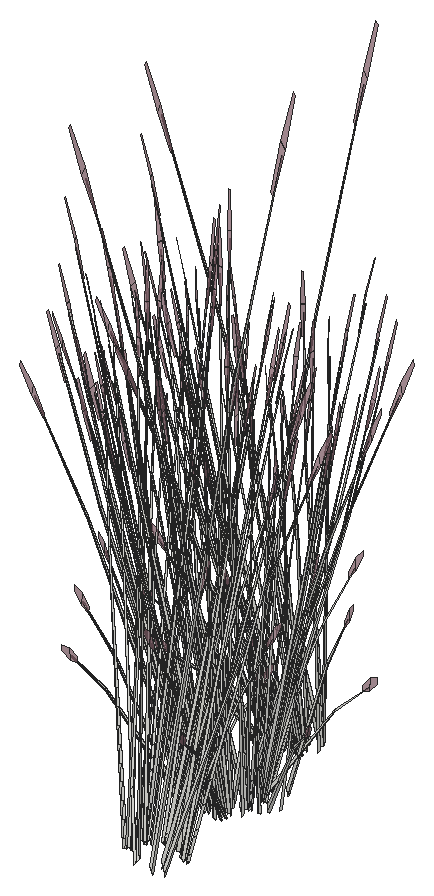
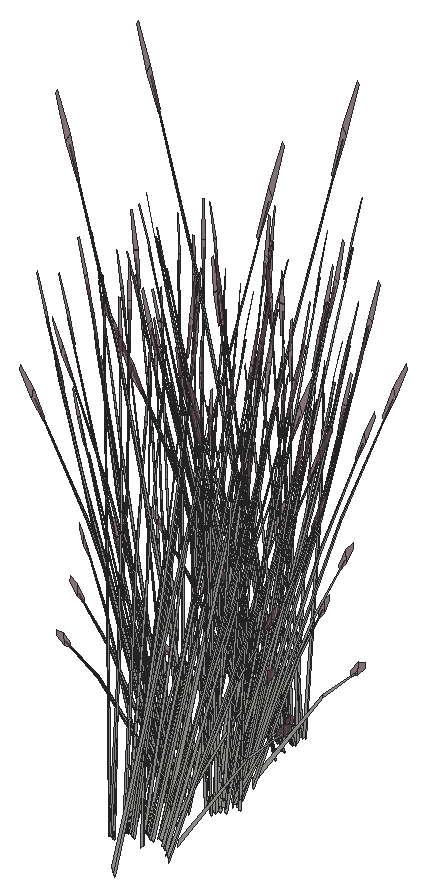
# SketchUp Ruby script. Lengths in inches.
U = 1.inch
M = Sketchup.active_model
def pt(a) = Geom::Point3d.new(a.map { |v| v * U })
def face(e, loops, mat)
  f = e.add_face(loops[0].map { |a| pt(a) })
  loops[1..].each { |l| e.add_face(l.map { |a| pt(a) }).erase! }
  f.material = f.back_material = mat if mat
  f
end
# faces: each face lists its corners as indices into pts; further lists are holes
def faces(e, pts, list, mat = nil) = list.each { |f| face(e, (f[0].is_a?(Array) ? f : [f]).map { |l| l.map { |i| pts[i] } }, mat) }
# xy, xz, yz: faces in a plane at the given z, y or x. An outline is a flat list of corners, or four numbers for a rectangle; further outlines are holes
def ring(l) = l.size == 4 ? [[l[0], l[1]], [l[2], l[1]], [l[2], l[3]], [l[0], l[3]]] : l.each_slice(2).to_a
def flat(e, list, mat, &to3) = list.each { |f| face(e, (f[0].is_a?(Array) ? f : [f]).map { |l| ring(l).map { |u, v| to3.(u, v) } }, mat) }
def xy(e, z, list, mat = nil) = flat(e, list, mat) { |x, y| [x, y, z] }
def xz(e, y, list, mat = nil) = flat(e, list, mat) { |x, z| [x, y, z] }
def yz(e, x, list, mat = nil) = flat(e, list, mat) { |y, z| [x, y, z] }
def lines(e, pts, list) = list.each { |a, b| e.add_line(pt(pts[a]), pt(pts[b])) }
# prism: a flat outline (further loops are holes) pulled along v
def prism(e, loops, v, mat = nil)
  f = face(e, loops, mat); d = Geom::Vector3d.new(v.map { |x| x * U })
  f.pushpull(f.normal.samedirection?(d) ? d.length : -d.length)
end
def box(e, o, s, mat = nil) = prism(e, [[o, [o[0] + s[0], o[1], o[2]], [o[0] + s[0], o[1] + s[1], o[2]], [o[0], o[1] + s[1], o[2]]]], [0, 0, s[2]], mat)
def at(x, y, z, deg = 0) = Geom::Transformation.translation(pt([x, y, z])) * Geom::Transformation.rotation(ORIGIN, Z_AXIS, deg.degrees)
def axes(o, x, y, z) = Geom::Transformation.new([*x, 0, *y, 0, *z, 0, *pt(o).to_a, 1])
def part(name) = M.definitions.add(name)
# library, detail: a bought-in or finely detailed component or shape, given as its bounding box
def library(name, o, s) = part(name).tap { |d| box(d.entities, o, s) }
def detail(e, o, s) = box(e.add_group.entities, o, s)
def put(e, d, t, mat = nil) = e.add_instance(d, t).tap { |i| i.material = mat if mat }
def group(e, t, mat = nil) = e.add_group.tap { |g| g.transformation = t; g.material = mat if mat }.entities
root = M.entities
M.materials.add("LightPink_Translucent").color = [144, 107, 117]
M.materials["LightPink_Translucent"].alpha = 0.75
c1 = part("blade")
p = [[2.15,0.21,22],[0,0.17,0],[0.09,0.45,0],[2.18,0.31,22],[2.29,0.31,22],[0.38,0.45,0],
  [2.48,0.24,33],[2.49,0.24,33],[2.48,0.22,33]]
faces(c1.entities,p,[[0,1,2,3],[4,5,2,3],[6,3,4,7],[8,0,3,6]])
c2 = part("seeds")
p = [[0.3,-0.1,1.38],[-0.01,-0.03,1.59],[-0.01,-0.03,0.03],[0.14,-0.07,-0.07],[0.29,-0.03,3],[0.15,0.01,3.11]]
faces(c2.entities,p,[[0,1,2,3],[1,0,4,5]],"LightPink_Translucent")
c3 = part("blade with seeds")
put(c3.entities,c1,at(0,0,0))
put(c3.entities,c2,axes([2.4,0.25,30.99],[1.5799,-0.05474,1.17369],[-0.12525,1.92788,0.29478],[-0.07173,-0.02425,1.56792]))
put(root,c3,axes([430.69,389.83,153.82],[0.23317,0.29531,-0.29918],[-0.26625,0.27955,0.38624],[0.13527,0.04253,0.73904]))
put(root,c3,axes([430.57,389.94,154],[-0.02064,0.35866,0.05432],[-0.3116,-0.00983,0.42765],[0.11936,0.03753,0.65209]))
put(root,c3,axes([428,395.12,154.21],[-0.19559,-0.38351,-0.60019],[0.40262,-0.21373,0.07243],[-0.04574,-0.1853,0.84903]))
put(root,c3,axes([427.23,389.3,153.82],[-0.35672,0.06741,-0.29918],[-0.09419,-0.38534,0.38624],[-0.10222,0.1035,0.73904]))
put(root,c3,axes([430.6,389.83,154],[-0.30217,0.31079,0.40553],[-0.2606,-0.33005,0.33437],[0.14177,0.05733,0.83914]))
put(root,c3,axes([428.8125,395.49,154.21],[0.01066,-0.43628,-0.60019],[0.44902,0.0293,0.07243],[0.04739,-0.18483,0.84903]))
put(root,c3,axes([429.4375,394.8125,153.98],[-0.00396,-0.09387,1.47793],[-0.33411,-0.2713,-0.23373],[0.05166,-0.16446,0.11853]))
put(root,c3,axes([428.03,394.79,153.82],[0.12355,-0.36271,-0.29918],[0.36044,0.10579,0.38624],[-0.03305,-0.14603,0.73904]))
put(root,c3,axes([428.31,395.27,153.27],[-0.0763,0.16212,1.44779],[-0.3201,-0.3355,0.11706],[0.1444,-0.2091,0.61892]))
put(root,c3,axes([429.35,394.48,153.98],[-0.04162,0.03603,1.49853],[-0.40776,-0.12155,-0.1416],[-0.01476,-0.15722,0.26519]))
put(root,c3,axes([429.86,389.07,153.27],[-0.15222,-0.08126,1.44779],[0.31502,-0.34091,0.11706],[0.19634,0.15379,0.61892]))
put(root,c3,axes([429.88,388,153.78],[-0.35411,-0.24507,1.16821],[0.37391,-0.38156,0.50405],[0.11425,0.22994,1.12919]))
put(root,c3,axes([427.85,395.04,153.95],[-0.40284,-0.11824,-0.43168],[0.13808,-0.40538,-0.33437],[-0.03694,-0.16321,0.82598]))
put(root,c3,axes([427.33,389.04,154.25],[0.37908,0.26007,-0.10273],[-0.21839,0.37663,-0.57019],[-0.1071,0.13092,0.8664]))
put(root,c3,axes([429.61,390.39,154.25],[0.2442,-0.40372,-0.10273],[0.35364,0.23259,-0.57019],[0.12293,0.11406,0.8664]))
put(root,c3,axes([428.72,395.35,153.95],[-0.29336,-0.31691,-0.43168],[0.3099,-0.27755,-0.33437],[0.04464,-0.16102,0.82598]))
put(root,c3,axes([427.13,393.78,153.98],[-0.00765,0.05653,1.49853],[-0.37706,0.20517,-0.1416],[-0.11096,-0.10488,0.26519]))
put(root,c3,axes([427.84,388.92,153.27],[0.10236,-0.14492,1.44779],[0.25844,0.39118,0.11706],[-0.17726,0.17814,0.61892]))
put(root,c3,axes([427.52,389.35,153.95],[0.10528,0.43067,-0.43168],[-0.39868,0.07534,-0.33437],[-0.11425,0.11568,0.82598]))
put(root,c3,axes([429.29,390.72,153.98],[0.00121,-0.0571,1.49853],[0.35119,-0.25193,-0.1416],[0.12199,0.08992,0.26519]))
put(root,c3,axes([427.75,390.07,154],[-0.33677,-0.02198,0.05432],[0.00923,-0.33185,0.42765],[-0.03524,0.12712,0.65209]))
put(root,c3,axes([428.19,395.02,154.25],[-0.40102,0.2196,-0.10273],[-0.19707,-0.38974,-0.57019],[-0.05291,-0.16424,0.8664]))
put(root,c3,axes([429.03,395.52,154.25],[-0.45039,-0.02337,-0.10273],[0.01231,-0.44247,-0.57019],[0.03129,-0.17041,0.8664]))
put(root,c3,axes([427.85,390.1,154],[-0.29182,-0.32181,0.40553],[0.3099,-0.27755,0.33437],[-0.05383,0.15098,0.83914]))
put(root,c3,axes([429.9,390.18,153.95],[0.40438,-0.11212,-0.43168],[0.07074,0.4246,-0.33437],[0.10862,0.12168,0.82598]))
put(root,c3,axes([429,395.23,153.82],[0.27728,-0.24833,-0.29918],[0.26248,0.28355,0.38624],[0.03994,-0.14407,0.73904]))
put(root,c3,axes([428.19,394.85,154],[0.30197,-0.1603,0.05432],[0.1478,0.29231,0.42765],[-0.02916,-0.12885,0.65209]))
put(root,c3,axes([427.12,395.23,154.21],[-0.34944,-0.22798,-0.60019],[0.24834,-0.39949,0.07243],[-0.1266,-0.13612,0.84903]))
put(root,c3,axes([426.99,394.93,153.82],[-0.06329,-0.37991,-0.29918],[0.36182,-0.10032,0.38624],[-0.09718,-0.10887,0.73904]))
put(root,c3,axes([429.7,390.53,154],[-0.18625,0.29962,0.05432],[-0.26523,-0.17444,0.42765],[0.08575,0.09606,0.65209]))
put(root,c3,axes([427.15,394.89,154],[0.18625,-0.29962,0.05432],[0.26523,0.17444,0.42765],[-0.08575,-0.09606,0.65209]))
put(root,c3,axes([429.78,390.45,154],[-0.4076,0.10824,0.40553],[-0.07074,-0.4246,0.33437],[0.09586,0.12514,0.83914]))
put(root,c3,axes([426.22,395.48,153.27],[0.15222,0.08126,1.44779],[-0.31502,0.34091,0.11706],[-0.19634,-0.15379,0.61892]))
put(root,c3,axes([427.77,389.28,153.27],[0.0763,-0.16212,1.44779],[0.3201,0.3355,0.11706],[-0.1444,0.2091,0.61892]))
put(root,c3,axes([428.66,390.58,154],[-0.30197,0.1603,0.05432],[-0.1478,-0.29231,0.42765],[0.02916,0.12885,0.65209]))
put(root,c3,axes([427.85,390.19,153.82],[-0.27728,0.24833,-0.29918],[-0.26248,-0.28355,0.38624],[-0.03994,0.14407,0.73904]))
put(root,c3,axes([426.9,390.12,153.98],[-0.01019,0.09334,1.47793],[0.28908,0.3247,-0.23373],[-0.07568,0.15355,0.11853]))
put(root,c3,axes([426.95,395.24,153.95],[-0.40438,0.11212,-0.43168],[-0.07074,-0.4246,-0.33437],[-0.10862,-0.12168,0.82598]))
put(root,c3,axes([427.82,389.91,154.56],[0.45039,0.02337,-0.11403],[-0.01231,0.44247,-0.63292],[-0.03129,0.17041,0.9617]))
put(root,c3,axes([428.66,390.4,154.25],[0.40102,-0.2196,-0.10273],[0.19707,0.38974,-0.57019],[0.05291,0.16424,0.8664]))
put(root,c3,axes([427.23,394.86,154.59],[-0.2735,0.45217,-0.11506],[-0.39608,-0.2605,-0.63862],[-0.13768,-0.12775,0.97037]))
put(root,c3,axes([429.1,395.36,154],[0.33677,0.02198,0.05432],[-0.00923,0.33185,0.42765],[0.03524,-0.12712,0.65209]))
put(root,c3,axes([429.34,396.25,154.21],[0.21406,-0.37215,-0.60019],[0.37511,0.26448,0.07243],[0.12781,-0.13483,0.84903]))
put(root,c3,axes([429.33,396.08,153.95],[-0.10528,-0.43067,-0.43168],[0.39868,-0.07534,-0.33437],[0.11425,-0.11568,0.82598]))
put(root,c3,axes([428.13,390.07,154.23],[0.29336,0.31691,-0.47917],[-0.3099,0.27755,-0.37115],[-0.04464,0.16102,0.91684]))
put(root,c3,axes([426.1875,394.73,153.98],[-0.08817,-0.00333,1.47793],[-0.28072,0.33293,-0.23373],[-0.14978,-0.06803,0.11853]))
put(root,c3,axes([429.52,396.39,154.25],[-0.37908,-0.26007,-0.10273],[0.21839,-0.37663,-0.57019],[0.1071,-0.13092,0.8664]))
put(root,c3,axes([429,390.38,153.95],[0.40284,0.11824,-0.43168],[-0.13808,0.40538,-0.33437],[0.03694,0.16321,0.82598]))
put(root,c3,axes([429.23,389.55,153.27],[-0.09368,-0.15143,1.44779],[0.43286,-0.12749,0.11706],[0.09783,0.23774,0.61892]))
put(root,c3,axes([427.95,397.81,152.81],[0.35414,0.19019,1.27785],[-0.34693,0.40974,0.50532],[-0.1554,-0.24285,1.07126]))
put(root,c3,axes([428.82,390.63,153.82],[-0.12355,0.36271,-0.29918],[-0.36044,-0.10579,0.38624],[0.03305,0.14603,0.73904]))
put(root,c3,axes([428.04,389.93,154.51],[-0.01066,0.43628,-0.66621],[-0.44902,-0.0293,0.0804],[-0.04739,0.18483,0.94242]))
put(root,c3,axes([430.45,396.27,153.98],[-0.05353,-0.00358,1.49853],[-0.22227,-0.38383,-0.1416],[0.08926,-0.1262,0.26519]))
put(root,c3,axes([426.87,391.08,153.98],[0.04649,-0.02848,1.49853],[0.38427,0.18941,-0.1416],[-0.00903,0.15771,0.26519]))
put(root,c3,axes([428.46,389.62,153.27],[-0.01003,-0.18103,1.44779],[0.43473,0.12009,0.11706],[-0.02689,0.25798,0.61892]))
put(root,c3,axes([429.625,396.125,153.82],[0.35672,-0.06741,-0.29918],[0.09419,0.38534,0.38624],[0.10222,-0.1035,0.73904]))
put(root,c3,axes([428.85,390.31,154.21],[0.19559,0.38351,-0.60019],[-0.40262,0.21373,0.07243],[0.04574,0.1853,0.84903]))
put(root,c3,axes([426.28,395.48,154],[0.02064,-0.35866,0.05432],[0.3116,0.00983,0.42765],[-0.11936,-0.03753,0.65209]))
put(root,c3,axes([426.16,395.59,153.82],[-0.23317,-0.29531,-0.29918],[0.26625,-0.27955,0.38624],[-0.13527,-0.04253,0.73904]))
put(root,c3,axes([428.5625,391.27,153.98],[0.05195,0.07595,1.47793],[0.41921,0.02984,-0.23373],[0.04216,0.1675,0.11853]))
put(root,c3,axes([426.4,395.79,154.21],[-0.40965,-0.01136,-0.60019],[0.02751,-0.47821,0.07243],[-0.17355,-0.05047,0.84903]))
put(root,c3,axes([427.89,390.54,152.84],[0.009,-0.24349,1.30391],[0.40497,0.12861,0.18019],[-0.03509,0.2595,0.61571]))
put(root,c3,axes([429.66,396.29,154],[0.28133,0.19836,0.05432],[-0.16379,0.28248,0.42765],[0.0902,-0.09132,0.65209]))
put(root,c3,axes([430.65,396.73,153.98],[0.05687,-0.07184,1.47793],[-0.07279,-0.44069,-0.23373],[0.14268,-0.08356,0.11853]))
put(root,c3,axes([425.85,395.01,153.98],[0.03038,0.04707,1.49853],[-0.14646,0.42312,-0.1416],[-0.14833,0.00306,0.26519]))
put(root,c3,axes([426.27,395.89,153.95],[-0.29757,0.31243,-0.43168],[-0.2606,-0.33005,-0.33437],[-0.15119,-0.04754,0.82598]))
put(root,c3,axes([426.42,395.56,154.25],[-0.02194,0.47967,-0.10273],[-0.41546,-0.01311,-0.57019],[-0.16001,-0.03332,0.8664]))
put(root,c3,axes([429.53,397.4,154.25],[-0.20619,-0.42709,-0.10273],[0.36595,-0.20988,-0.57019],[0.15422,-0.05635,0.8664]))
put(root,c3,axes([429.51,397.03,153.95],[0.11102,-0.42903,-0.43168],[0.38064,0.14706,-0.33437],[0.15325,-0.03934,0.82598]))
put(root,c3,axes([425.89,396.22,153.27],[0.16998,-0.01068,1.44779],[-0.11276,0.46299,0.11706],[-0.24224,-0.02864,0.61892]))
put(root,c3,axes([429.44,397.19,154.21],[0.3601,-0.20831,-0.60019],[0.20068,0.4288,0.07243],[0.17399,-0.04871,0.84903]))
put(root,c3,axes([425.8,396.46,154],[-0.15051,-0.3216,0.05432],[0.27447,-0.15741,0.42765],[-0.12099,0.03106,0.65209]))
put(root,c3,axes([429.75,397.23,153.82],[0.34057,0.13158,-0.29918],[-0.09933,0.38387,0.38624],[0.13712,-0.0352,0.73904]))
put(root,c3,axes([425.74,396.62,153.82],[-0.34057,-0.13158,-0.29918],[0.09933,-0.38387,0.38624],[-0.13712,0.0352,0.73904]))
put(root,c3,axes([428.82,396.75,153.27],[-0.16998,0.01068,1.44779],[0.11276,-0.46299,0.11706],[0.24224,0.02864,0.61892]))
put(root,c3,axes([429.7,397.39,154],[0.15051,0.3216,0.05432],[-0.27447,0.15741,0.42765],[0.12099,-0.03106,0.65209]))
put(root,c3,axes([426.78,396.55,152.82],[0.11649,-0.06823,1.49584],[0.04017,0.47639,0.11706],[-0.25231,0.06321,0.53462]))
put(root,c3,axes([430.35,398.67,153.98],[-0.03706,-0.04129,1.49853],[0.08106,-0.44261,-0.1416],[0.14596,-0.02828,0.26519]))
put(root,c3,axes([425.53,396.875,153.98],[-0.06692,0.06124,1.47793],[0.00569,0.44742,-0.23373],[-0.15339,0.05818,0.11853]))
put(root,c3,axes([425.98,396.8125,153.95],[-0.11102,0.42903,-0.43168],[-0.38064,-0.14706,-0.33437],[-0.15325,0.03934,0.82598]))
put(root,c3,axes([425.96,396.45,154.25],[0.20619,0.42709,-0.10273],[-0.36595,0.20988,-0.57019],[-0.15422,0.05635,0.8664]))
put(root,c3,axes([430.03,398.3,153.32],[-0.07843,-0.39649,-0.0295],[0.37072,-0.09115,-0.13375],[0.07742,0.02514,0.44114]))
put(root,c3,axes([429.07,398.29,154.25],[0.02194,-0.47967,-0.10273],[0.41546,0.01311,-0.57019],[0.16001,0.03332,0.8664]))
put(root,c3,axes([425.76,402.58,153.27],[0.09368,0.15143,1.44779],[-0.43286,0.12749,0.11706],[-0.09783,-0.23774,0.61892]))
put(root,c3,axes([426.47,401.58,153.98],[-0.06268,-0.06613,1.47793],[-0.4183,0.04193,-0.23373],[-0.06676,-0.15817,0.11853]))
put(root,c3,axes([426.91,402.7,154.21],[-0.19559,-0.38351,-0.60019],[0.40262,-0.21373,0.07243],[-0.04574,-0.1853,0.84903]))
put(root,c3,axes([429.43,398,153.98],[0.08791,-0.00798,1.47793],[0.24113,-0.36643,-0.23373],[0.15637,0.04837,0.11853]))
put(root,c3,axes([425.84,397.56,154],[-0.28133,-0.19836,0.05432],[0.16379,-0.28248,0.42765],[-0.0902,0.09132,0.65209]))
put(root,c3,axes([425.97,397.04,153.27],[0.14219,-0.09977,1.44779],[0.11971,0.461,0.11706],[-0.22323,0.10419,0.61892]))
put(root,c3,axes([429.09,398.06,154.21],[0.40965,0.01136,-0.60019],[-0.02751,0.47821,0.07243],[0.17355,0.05047,0.84903]))
put(root,c3,axes([427.73,403.07,154.21],[0.01066,-0.43628,-0.60019],[0.44902,0.0293,0.07243],[0.04739,-0.18483,0.84903]))
put(root,c3,axes([428.35,402.39,153.98],[-0.00396,-0.09387,1.47793],[-0.33411,-0.2713,-0.23373],[0.05166,-0.16446,0.11853]))
put(root,c3,axes([426.95,402.37,153.82],[0.12355,-0.36271,-0.29918],[0.36044,0.10579,0.38624],[-0.03305,-0.14603,0.73904]))
put(root,c3,axes([427.22,402.85,153.27],[-0.0763,0.16212,1.44779],[-0.3201,-0.3355,0.11706],[0.1444,-0.2091,0.61892]))
put(root,c3,axes([428.26,402.05,153.98],[-0.04162,0.03603,1.49853],[-0.40776,-0.12155,-0.1416],[-0.01476,-0.15722,0.26519]))
put(root,c3,axes([426.77,402.62,153.95],[-0.40284,-0.11824,-0.43168],[0.13808,-0.40538,-0.33437],[-0.03694,-0.16321,0.82598]))
put(root,c3,axes([424.79,397.33,153.98],[0.0523,0.01265,1.49853],[0.16179,0.41674,-0.1416],[-0.10706,0.10938,0.26519]))
put(root,c3,axes([427.64,402.93,153.95],[-0.29336,-0.31691,-0.43168],[0.3099,-0.27755,-0.33437],[0.04464,-0.16102,0.82598]))
put(root,c3,axes([429.34,398.26,153.82],[0.23317,0.29531,-0.29918],[-0.26625,0.27955,0.38624],[0.13527,0.04253,0.73904]))
put(root,c3,axes([429.22,398.37,154],[-0.02064,0.35866,0.05432],[-0.3116,-0.00983,0.42765],[0.11936,0.03753,0.65209]))
put(root,c3,axes([426.04,401.36,153.98],[-0.00765,0.05653,1.49853],[-0.37706,0.20517,-0.1416],[-0.11096,-0.10488,0.26519]))
put(root,c3,axes([425.87,397.73,153.82],[-0.35672,0.06741,-0.29918],[-0.09419,-0.38534,0.38624],[-0.10222,0.1035,0.73904]))
put(root,c3,axes([427.11,402.6,154.25],[-0.40102,0.2196,-0.10273],[-0.19707,-0.38974,-0.57019],[-0.05291,-0.16424,0.8664]))
put(root,c3,axes([427.94,403.09,154.25],[-0.45039,-0.02337,-0.10273],[0.01231,-0.44247,-0.57019],[0.03129,-0.17041,0.8664]))
put(root,c3,axes([427.91,402.81,153.82],[0.27728,-0.24833,-0.29918],[0.26248,0.28355,0.38624],[0.03994,-0.14407,0.73904]))
put(root,c3,axes([427.1,402.42,154],[0.30197,-0.1603,0.05432],[0.1478,0.29231,0.42765],[-0.02916,-0.12885,0.65209]))
put(root,c3,axes([426.03,402.81,154.21],[-0.34944,-0.22798,-0.60019],[0.24834,-0.39949,0.07243],[-0.1266,-0.13612,0.84903]))
put(root,c3,axes([425.91,402.5,153.82],[-0.06329,-0.37991,-0.29918],[0.36182,-0.10032,0.38624],[-0.09718,-0.10887,0.73904]))
put(root,c3,axes([428.5,397.5,153.27],[-0.15222,-0.08126,1.44779],[0.31502,-0.34091,0.11706],[0.19634,0.15379,0.61892]))
put(root,c3,axes([428.53,396.43,153.78],[-0.35411,-0.24507,1.16821],[0.37391,-0.38156,0.50405],[0.11425,0.22994,1.12919]))
put(root,c3,axes([425.98,397.46,154.25],[0.37908,0.26007,-0.10273],[-0.21839,0.37663,-0.57019],[-0.1071,0.13092,0.8664]))
put(root,c3,axes([426.07,402.47,154],[0.18625,-0.29962,0.05432],[0.26523,0.17444,0.42765],[-0.08575,-0.09606,0.65209]))
put(root,c3,axes([428.25,398.81,154.25],[0.2442,-0.40372,-0.10273],[0.35364,0.23259,-0.57019],[0.12293,0.11406,0.8664]))
put(root,c3,axes([426.49,397.35,153.27],[0.10236,-0.14492,1.44779],[0.25844,0.39118,0.11706],[-0.17726,0.17814,0.61892]))
put(root,c3,axes([425.13,403.06,153.27],[0.15222,0.08126,1.44779],[-0.31502,0.34091,0.11706],[-0.19634,-0.15379,0.61892]))
put(root,c3,axes([426.16,397.77,153.95],[0.10528,0.43067,-0.43168],[-0.39868,0.07534,-0.33437],[-0.11425,0.11568,0.82598]))
put(root,c3,axes([427.93,399.15,153.98],[0.00121,-0.0571,1.49853],[0.35119,-0.25193,-0.1416],[0.12199,0.08992,0.26519]))
put(root,c3,axes([425.87,402.82,153.95],[-0.40438,0.11212,-0.43168],[-0.07074,-0.4246,-0.33437],[-0.10862,-0.12168,0.82598]))
put(root,c3,axes([426.39,398.49,154],[-0.33677,-0.02198,0.05432],[0.00923,-0.33185,0.42765],[-0.03524,0.12712,0.65209]))
put(root,c3,axes([426.15,402.4375,154.59],[-0.2735,0.45217,-0.11506],[-0.39608,-0.2605,-0.63862],[-0.13768,-0.12775,0.97037]))
put(root,c3,axes([428.02,402.9375,154],[0.33677,0.02198,0.05432],[-0.00923,0.33185,0.42765],[0.03524,-0.12712,0.65209]))
put(root,c3,axes([428.54,398.61,153.95],[0.40438,-0.11212,-0.43168],[0.07074,0.4246,-0.33437],[0.10862,0.12168,0.82598]))
put(root,c3,axes([428.26,403.83,154.21],[0.21406,-0.37215,-0.60019],[0.37511,0.26448,0.07243],[0.12781,-0.13483,0.84903]))
put(root,c3,axes([428.24,403.66,153.95],[-0.10528,-0.43067,-0.43168],[0.39868,-0.07534,-0.33437],[0.11425,-0.11568,0.82598]))
put(root,c3,axes([428.34,398.96,154],[-0.18625,0.29962,0.05432],[-0.26523,-0.17444,0.42765],[0.08575,0.09606,0.65209]))
put(root,c3,axes([425.1,402.31,153.98],[-0.08817,-0.00333,1.47793],[-0.28072,0.33293,-0.23373],[-0.14978,-0.06803,0.11853]))
put(root,c3,axes([428.43,403.96,154.25],[-0.37908,-0.26007,-0.10273],[0.21839,-0.37663,-0.57019],[0.1071,-0.13092,0.8664]))
put(root,c3,axes([426.41,397.7,153.27],[0.0763,-0.16212,1.44779],[0.3201,0.3355,0.11706],[-0.1444,0.2091,0.61892]))
put(root,c3,axes([426.87,405.38,152.81],[0.35414,0.19019,1.27785],[-0.34693,0.40974,0.50532],[-0.1554,-0.24285,1.07126]))
